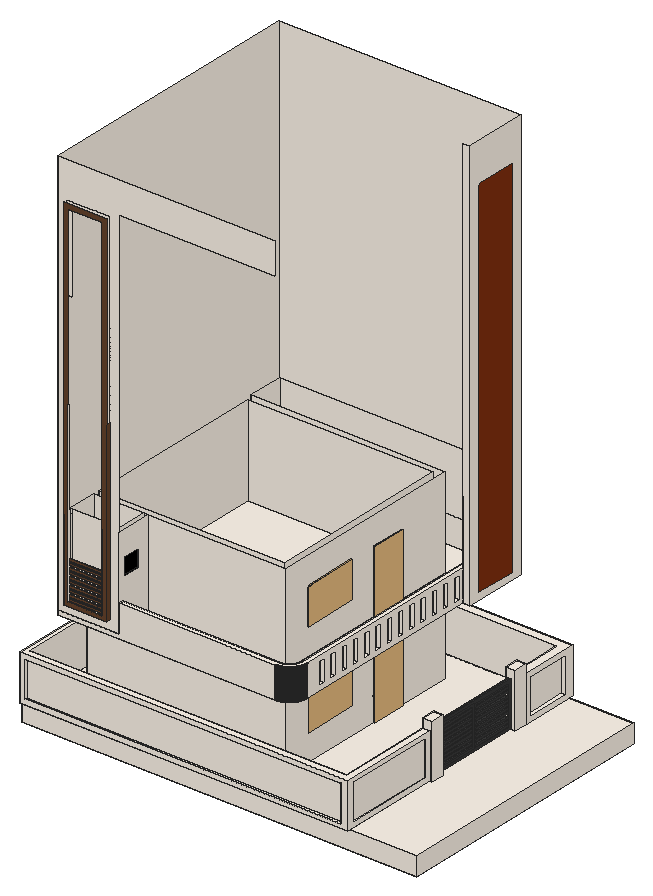
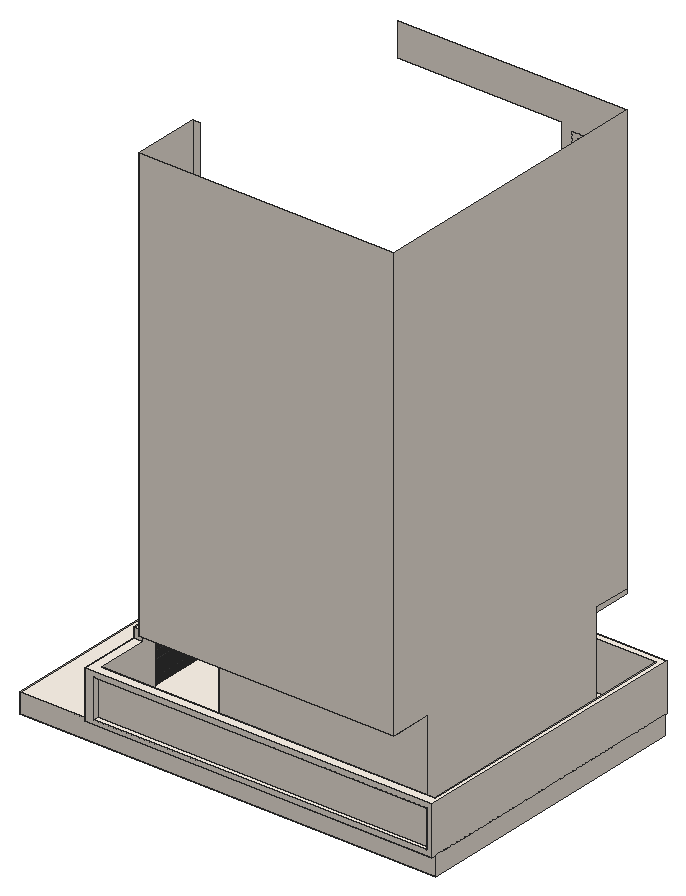
# SketchUp Ruby script. Lengths in inches.
U = 1.inch
M = Sketchup.active_model
def pt(a) = Geom::Point3d.new(a.map { |v| v * U })
def face(e, loops, mat)
  f = e.add_face(loops[0].map { |a| pt(a) })
  loops[1..].each { |l| e.add_face(l.map { |a| pt(a) }).erase! }
  f.material = f.back_material = mat if mat
  f
end
# faces: each face lists its corners as indices into pts; further lists are holes
def faces(e, pts, list, mat = nil) = list.each { |f| face(e, (f[0].is_a?(Array) ? f : [f]).map { |l| l.map { |i| pts[i] } }, mat) }
# xy, xz, yz: faces in a plane at the given z, y or x. An outline is a flat list of corners, or four numbers for a rectangle; further outlines are holes
def ring(l) = l.size == 4 ? [[l[0], l[1]], [l[2], l[1]], [l[2], l[3]], [l[0], l[3]]] : l.each_slice(2).to_a
def flat(e, list, mat, &to3) = list.each { |f| face(e, (f[0].is_a?(Array) ? f : [f]).map { |l| ring(l).map { |u, v| to3.(u, v) } }, mat) }
def xy(e, z, list, mat = nil) = flat(e, list, mat) { |x, y| [x, y, z] }
def xz(e, y, list, mat = nil) = flat(e, list, mat) { |x, z| [x, y, z] }
def yz(e, x, list, mat = nil) = flat(e, list, mat) { |y, z| [x, y, z] }
def lines(e, pts, list) = list.each { |a, b| e.add_line(pt(pts[a]), pt(pts[b])) }
# prism: a flat outline (further loops are holes) pulled along v
def prism(e, loops, v, mat = nil)
  f = face(e, loops, mat); d = Geom::Vector3d.new(v.map { |x| x * U })
  f.pushpull(f.normal.samedirection?(d) ? d.length : -d.length)
end
def box(e, o, s, mat = nil) = prism(e, [[o, [o[0] + s[0], o[1], o[2]], [o[0] + s[0], o[1] + s[1], o[2]], [o[0], o[1] + s[1], o[2]]]], [0, 0, s[2]], mat)
def at(x, y, z, deg = 0) = Geom::Transformation.translation(pt([x, y, z])) * Geom::Transformation.rotation(ORIGIN, Z_AXIS, deg.degrees)
def axes(o, x, y, z) = Geom::Transformation.new([*x, 0, *y, 0, *z, 0, *pt(o).to_a, 1])
def part(name) = M.definitions.add(name)
# library, detail: a bought-in or finely detailed component or shape, given as its bounding box
def library(name, o, s) = part(name).tap { |d| box(d.entities, o, s) }
def detail(e, o, s) = box(e.add_group.entities, o, s)
def put(e, d, t, mat = nil) = e.add_instance(d, t).tap { |i| i.material = mat if mat }
def group(e, t, mat = nil) = e.add_group.tap { |g| g.transformation = t; g.material = mat if mat }.entities
root = M.entities
M.materials.add("C01_Vanilla_Cream").color = [255, 246, 235]
M.materials.add("Hardwood_Double_Herringbone_4K").color = [130, 48, 16]
M.materials.add("M07_Charcoal_Gleam").color = [58, 58, 58]
M.materials.add("Wood_Veneer_15_1K").color = [103, 69, 45]
M.materials.add("[Color_009]1").color = [0, 0, 0]
c1 = library("porta+4",[0.2,-5.42,1.33],[46.55,4.72,83.21])
c2 = library("mesh-164",[-1582.71,-3144.16,-23.22],[2366.42,2227.34,65.81])
c3 = part("Group13")
put(c3.entities,c2,at(294.66,859.51,3.5))
xy(root,0,[[0,6,523.6875,366]],"C01_Vanilla_Cream")
xy(root,24,[[0,3,435,6],[[0,6,0,366,438,366,438,276.27,432,276.27,432,156.27,438,156.27,438,138.27,435,138.27,435,6],[6,12,426,12,426,156.27,429,156.27,429,276.27,426,276.27,426,360,6,360]],[435,6,523.6875,6,523.6875,366,438,366,438,276.27,432,276.27,432,156.27,438,156.27,438,138.27,435,138.27],[[6,12,426,12,426,156.27,429,156.27,429,276.27,426,276.27,426,360,6,360],[48,54,312,318]],[57,63,303,309],
  [0,366,438,372.04]],"C01_Vanilla_Cream")
xy(root,27,[[303,201,312,243]],"C01_Vanilla_Cream")
xy(root,30,[[6,3,426,6],[432,12,435,132.27],[432,300.27,438,360],[6,366,426,372.04]],"C01_Vanilla_Cream")
xy(root,31.5,[[429,161.27,432,214.27],[429,218.27,432,271.27]],"M07_Charcoal_Gleam")
xy(root,34,[[429,161.27,432,214.27],[429,218.27,432,271.27]],"C01_Vanilla_Cream")
xy(root,36.5,[[429,161.27,432,214.27],[429,218.27,432,271.27]],"M07_Charcoal_Gleam")
xy(root,39,[[429,218.27,432,271.27]],"C01_Vanilla_Cream")
xy(root,39,[[429,161.27,432,214.27]],"M07_Charcoal_Gleam")
xy(root,41.5,[[429,161.27,432,214.27],[429,218.27,432,271.27]],"M07_Charcoal_Gleam")
xy(root,44,[[429,218.27,432,271.27]],"C01_Vanilla_Cream")
xy(root,44,[[429,161.27,432,214.27]],"M07_Charcoal_Gleam")
xy(root,46.5,[[429,161.27,432,214.27],[429,218.27,432,271.27]],"M07_Charcoal_Gleam")
xy(root,49,[[429,161.27,432,214.27],[429,218.27,432,271.27]],"M07_Charcoal_Gleam")
xy(root,51.5,[[429,161.27,432,214.27],[429,218.27,432,271.27]],"M07_Charcoal_Gleam")
xy(root,54,[[429,161.27,432,214.27],[429,218.27,432,271.27]],"M07_Charcoal_Gleam")
xy(root,56.5,[[429,161.27,432,214.27],[429,218.27,432,271.27]],"M07_Charcoal_Gleam")
xy(root,59,[[429,161.27,432,214.27],[429,218.27,432,271.27]],"M07_Charcoal_Gleam")
xy(root,61.5,[[429,161.27,432,214.27],[429,218.27,432,271.27]],"M07_Charcoal_Gleam")
xy(root,63,[[303,93,312,159]],"C01_Vanilla_Cream")
xy(root,64,[[429,161.27,432,214.27],[429,218.27,432,271.27]],"M07_Charcoal_Gleam")
xy(root,66.5,[[429,161.27,432,214.27],[429,218.27,432,271.27]],"M07_Charcoal_Gleam")
xy(root,69,[[429,161.27,432,214.27],[429,218.27,432,271.27]],"M07_Charcoal_Gleam")
xy(root,71.5,[[429,161.27,432,214.27],[429,218.27,432,271.27]],"M07_Charcoal_Gleam")
xy(root,74,[[429,161.27,432,214.27],[429,218.27,432,271.27]],"M07_Charcoal_Gleam")
xy(root,76.5,[[429,161.27,432,214.27],[429,218.27,432,271.27]],"M07_Charcoal_Gleam")
xy(root,78,[[6,3,426,6],[432,12,435,132.27],[432,300.27,438,360],[6,366,426,372.04]],"C01_Vanilla_Cream")
xy(root,79,[[429,161.27,432,214.27],[429,218.27,432,271.27]],"M07_Charcoal_Gleam")
xy(root,84,[[0,3,435,3,435,138.27,426,138.27,426,12,6,12,6,360,426,360,426,294.27,438,294.27,438,372.04,0,372.04]],"C01_Vanilla_Cream")
xy(root,84,[[429,156.27,432,276.27]],"M07_Charcoal_Gleam")
xy(root,96,[[426,138.27,438,156.27],[426,276.27,438,294.27]],"C01_Vanilla_Cream")
xy(root,105,[[303,93,312,159],[303,201,312,243]],"C01_Vanilla_Cream")
xy(root,144,[[48,54,312,63],[57,63,303,309],[303,63,312,318],[360,288,360,366,48,366,48,372,369,372,369,288],[57,309,303,318],
  [48,318,57,366],[57,318,303,366],[303,318,312,366]],"C01_Vanilla_Cream")
xy(root,144,[[48,6,48,54,312,54,312,366,360,366,360,30,359.99,29.25,359.95,28.49,359.89,27.74,359.8125,26.99,359.7,26.25,359.57,25.5,359.42,24.76,359.25,24.03,359.05,23.3,358.83,22.58,358.58,21.87,358.31,21.17,358.03,20.47,357.72,19.78,357.38,19.1,357.03,18.4375,356.66,17.78,356.26,17.14,355.85,16.51,355.42,15.89,354.96,15.29,354.49,14.7,354,14.13,353.5,13.57,352.97,13.03,352.43,12.5,351.87,12,351.3,11.51,350.71,11.04,350.11,10.58,349.49,10.15,348.86,9.74,348.22,9.34,347.5625,8.97,346.9,8.62,346.22,8.28,345.53,7.97,344.83,7.69,344.13,7.42,343.42,7.17,342.7,6.95,341.97,6.75,341.24,6.58,340.5,6.43,339.75,6.3,339.01,6.1875,338.26,6.11,337.51,6.05,336.75,6.01,336,6]],"Wood_Veneer_15_1K")
xy(root,150,[[48,6,129,6,129,54,123,54,123,12,57,12,57,54,48,54],[129,12,336,12,336.57,12.01,337.13,12.04,337.69,12.08,338.26,12.14,338.82,12.22,339.37,12.32,339.93,12.43,340.48,12.57,341.02,12.71,341.5625,12.88,342.1,13.0625,342.625,13.26,343.15,13.48,343.66,13.71,344.17,13.96,344.67,14.23,345.16,14.51,345.64,14.8,346.12,15.11,346.58,15.4375,347.03,15.78,347.47,16.13,347.9,16.5,348.32,16.88,348.73,17.27,349.12,17.68,349.5,18.1,349.87,18.53,350.22,18.97,350.5625,19.42,350.89,19.88,351.2,20.36,351.49,20.84,351.77,21.33,352.04,21.83,352.29,22.34,352.52,22.85,352.74,23.375,352.9375,23.9,353.12,24.4375,353.29,24.98,353.43,25.52,353.57,26.07,353.68,26.63,353.78,27.18,353.86,27.74,353.92,28.31,353.96,28.87,353.99,29.43,354,30,354,366,54,366,54,318,312,318,312,54,129,54],[57,12,123,54],[354,48.59,360,57.93],[57,63,303,309],
  [354,67.26,360,76.6],[354,85.93,360,95.27],[354,104.61,360,113.94],[354,123.28,360,132.62],[354,141.95,360,151.29],
  [354,160.625,360,169.96],[354,179.3,360,188.64],[354,197.97,360,207.31],[354,216.64,360,225.98],[354,235.32,360,244.65],
  [354,253.99,360,263.33],[354,272.66,360,282]],"C01_Vanilla_Cream")
xy(root,153,[[303,201,312,243],[360,303,369,357]],"C01_Vanilla_Cream")
xy(root,162,[[60,0,117,6]],"Wood_Veneer_15_1K")
xy(root,168,[[66,0,111,6]],"C01_Vanilla_Cream")
xy(root,169,[[66,1,111,2]],"C01_Vanilla_Cream")
xy(root,171.68,[[66,1,111,2]],"C01_Vanilla_Cream")
xy(root,174.35,[[66,1,111,2]],"C01_Vanilla_Cream")
xy(root,177.03,[[66,1,111,2]],"C01_Vanilla_Cream")
xy(root,179.7,[[66,1,111,2]],"C01_Vanilla_Cream")
xy(root,180,[[354,48.59,360,57.93],[354,67.26,360,76.6],[354,85.93,360,95.27],[354,104.61,360,113.94],[354,123.28,360,132.62],
  [354,141.95,360,151.29],[354,160.625,360,169.96],[354,179.3,360,188.64],[354,197.97,360,207.31],[354,216.64,360,225.98],
  [354,235.32,360,244.65],[354,253.99,360,263.33],[354,272.66,360,282]],"C01_Vanilla_Cream")
xy(root,182.375,[[66,1,111,2]],"C01_Vanilla_Cream")
xy(root,185.05,[[66,1,111,2]],"C01_Vanilla_Cream")
xy(root,186,[[129,6,336,6,336.75,6.01,337.51,6.05,338.26,6.11,339.01,6.1875,339.75,6.3,340.5,6.43,341.24,6.58,341.97,6.75,342.7,6.95,343.42,7.17,344.13,7.42,344.83,7.69,345.53,7.97,346.22,8.28,346.9,8.62,347.5625,8.97,348.22,9.34,348.86,9.74,349.49,10.15,350.11,10.58,350.71,11.04,351.3,11.51,351.87,12,352.43,12.5,352.97,13.03,353.5,13.57,354,14.13,354.49,14.7,354.96,15.29,355.42,15.89,355.85,16.51,356.26,17.14,356.66,17.78,357.03,18.4375,357.38,19.1,357.72,19.78,358.03,20.47,358.31,21.17,358.58,21.87,358.83,22.58,359.05,23.3,359.25,24.03,359.42,24.76,359.57,25.5,359.7,26.25,359.8125,26.99,359.89,27.74,359.95,28.49,359.99,29.25,360,30,360,366,354,366,354,30,353.99,29.43,353.96,28.87,353.92,28.31,353.86,27.74,353.78,27.18,353.68,26.63,353.57,26.07,353.43,25.52,353.29,24.98,353.12,24.4375,352.9375,23.9,352.74,23.375,352.52,22.85,352.29,22.34,352.04,21.83,351.77,21.33,351.49,20.84,351.2,20.36,350.89,19.88,350.5625,19.42,350.22,18.97,349.87,18.53,349.5,18.1,349.12,17.68,348.73,17.27,348.32,16.88,347.9,16.5,347.47,16.13,347.03,15.78,346.58,15.4375,346.12,15.11,345.64,14.8,345.16,14.51,344.67,14.23,344.17,13.96,343.66,13.71,343.15,13.48,342.625,13.26,342.1,13.0625,341.5625,12.88,341.02,12.71,340.48,12.57,339.93,12.43,339.37,12.32,338.82,12.22,338.26,12.14,337.69,12.08,337.13,12.04,336.57,12.01,336,12,129,12]],"C01_Vanilla_Cream")
xy(root,187.73,[[66,1,111,2]],"C01_Vanilla_Cream")
xy(root,189,[[303,93,312,159]],"C01_Vanilla_Cream")
xy(root,190.4,[[66,1,111,2]],"C01_Vanilla_Cream")
xy(root,193.08,[[66,1,111,2]],"C01_Vanilla_Cream")
xy(root,195.75,[[66,1,111,2]],"C01_Vanilla_Cream")
xy(root,198.43,[[66,1,111,2]],"C01_Vanilla_Cream")
xy(root,201.1,[[66,1,111,2]],"C01_Vanilla_Cream")
xy(root,203.78,[[66,1,111,2]],"C01_Vanilla_Cream")
xy(root,206.45,[[66,1,111,2]],"C01_Vanilla_Cream")
xy(root,209.125,[[66,1,111,2]],"C01_Vanilla_Cream")
xy(root,211.8,[[66,1,111,2]],"C01_Vanilla_Cream")
xy(root,213.8,[[126,14.34,129,38.34]],"[Color_009]1")
xy(root,214.48,[[66,1,111,2]],"C01_Vanilla_Cream")
xy(root,217.15,[[66,1,111,2]],"C01_Vanilla_Cream")
xz(root,0,[[[60,162,117,642],[66,168,111,636]]],"Wood_Veneer_15_1K")
xz(root,1,[[66,169,111,171.68],[66,174.35,111,177.03],[66,179.7,111,182.375],[66,185.05,111,187.73],[66,190.4,111,193.08],
  [66,195.75,111,198.43],[66,201.1,111,203.78],[66,206.45,111,209.125],[66,211.8,111,214.48],[66,217.15,111,219.82]],"Wood_Veneer_15_1K")
xz(root,2,[[66,169,111,171.68],[66,174.35,111,177.03],[66,179.7,111,182.375],[66,185.05,111,187.73],[66,190.4,111,193.08],
  [66,195.75,111,198.43],[66,201.1,111,203.78],[66,206.45,111,209.125],[66,211.8,111,214.48],[66,217.15,111,219.82]],"C01_Vanilla_Cream")
xz(root,3,[[[0,24,435,84],[6,30,426,78]]],"C01_Vanilla_Cream")
xz(root,6,[[0,0,523.6875,24],[6,30,426,78],[48,144,336,144,336,186,129,186,129,150,48,150],[[48,150,129,150,129,648,336,648,336,690,48,690],[60,162,117,642]],[60,162,117,162,117,642,60,642,60,528,66,528,66,636,111,636,111,168,66,168,66,276,60,276],
  [66,168,111,276]],"C01_Vanilla_Cream")
xz(root,12,[[6,24,426,84],[432,30,435,78],[57,150,123,270],[129,150,135,186],[135,150,336,186]],"C01_Vanilla_Cream")
xz(root,14.34,[[126,213.8,129,237.8]],"[Color_009]1")
xz(root,38.34,[[126,213.8,129,237.8]],"[Color_009]1")
xz(root,48.59,[[354,150,360,180]],"C01_Vanilla_Cream")
xz(root,54,[[48,24,312,144],[48,144,57,150],[57,150,123,270],[123,150,129,270],[129,150,312,270]],"C01_Vanilla_Cream")
xz(root,57.93,[[354,150,360,180]],"C01_Vanilla_Cream")
xz(root,63,[[57,24,303,144],[57,150,303,270]],"C01_Vanilla_Cream")
xz(root,67.26,[[354,150,360,180]],"C01_Vanilla_Cream")
xz(root,76.6,[[354,150,360,180]],"C01_Vanilla_Cream")
xz(root,85.93,[[354,150,360,180]],"C01_Vanilla_Cream")
xz(root,93,[[303,63,312,105],[303,189,312,231]],"C01_Vanilla_Cream")
xz(root,95.27,[[354,150,360,180]],"C01_Vanilla_Cream")
xz(root,104.61,[[354,150,360,180]],"C01_Vanilla_Cream")
xz(root,113.94,[[354,150,360,180]],"C01_Vanilla_Cream")
xz(root,123.28,[[354,150,360,180]],"C01_Vanilla_Cream")
xz(root,132.27,[[432,30,435,78]],"C01_Vanilla_Cream")
xz(root,132.62,[[354,150,360,180]],"C01_Vanilla_Cream")
xz(root,138.27,[[435,24,438,24,438,96,426,96,426,84,435,84]],"C01_Vanilla_Cream")
xz(root,141.95,[[354,150,360,180]],"C01_Vanilla_Cream")
xz(root,151.29,[[354,150,360,180]],"C01_Vanilla_Cream")
xz(root,156.27,[[426,24,426,96,438,96,438,24,432,24,432,84,429,84,429,24]],"C01_Vanilla_Cream")
xz(root,159,[[303,63,312,105],[303,189,312,231]],"C01_Vanilla_Cream")
xz(root,160.625,[[354,150,360,180]],"C01_Vanilla_Cream")
xz(root,161.27,[[429,31.5,432,34],[429,36.5,432,39],[429,41.5,432,44],[429,46.5,432,49],[429,51.5,432,54],
  [429,56.5,432,59],[429,61.5,432,64],[429,66.5,432,69],[429,71.5,432,74],[429,76.5,432,79]],"C01_Vanilla_Cream")
xz(root,169.96,[[354,150,360,180]],"C01_Vanilla_Cream")
xz(root,179.3,[[354,150,360,180]],"C01_Vanilla_Cream")
xz(root,188.64,[[354,150,360,180]],"C01_Vanilla_Cream")
xz(root,197.97,[[354,150,360,180]],"C01_Vanilla_Cream")
xz(root,201,[[303,27,312,105],[303,153,312,231]],"C01_Vanilla_Cream")
xz(root,207.31,[[354,150,360,180]],"C01_Vanilla_Cream")
xz(root,214.27,[[429,31.5,432,34],[429,36.5,432,39],[429,41.5,432,44],[429,46.5,432,49],[429,51.5,432,54],
  [429,56.5,432,59],[429,61.5,432,64],[429,66.5,432,69],[429,71.5,432,74]],"C01_Vanilla_Cream")
xz(root,214.27,[[429,76.5,432,79]],"M07_Charcoal_Gleam")
xz(root,216.64,[[354,150,360,180]],"C01_Vanilla_Cream")
xz(root,218.27,[[429,31.5,432,34],[429,36.5,432,39],[429,41.5,432,44],[429,46.5,432,49],[429,51.5,432,54],
  [429,56.5,432,59],[429,61.5,432,64],[429,66.5,432,69],[429,71.5,432,74],[429,76.5,432,79]],"C01_Vanilla_Cream")
xz(root,225.98,[[354,150,360,180]],"C01_Vanilla_Cream")
xz(root,235.32,[[354,150,360,180]],"C01_Vanilla_Cream")
xz(root,243,[[303,27,312,105],[303,153,312,231]],"C01_Vanilla_Cream")
xz(root,244.65,[[354,150,360,180]],"C01_Vanilla_Cream")
xz(root,253.99,[[354,150,360,180]],"C01_Vanilla_Cream")
xz(root,263.33,[[354,150,360,180]],"C01_Vanilla_Cream")
xz(root,271.27,[[429,31.5,432,34],[429,36.5,432,39],[429,41.5,432,44],[429,46.5,432,49],[429,51.5,432,54],
  [429,56.5,432,59],[429,61.5,432,64],[429,66.5,432,69],[429,71.5,432,74],[429,76.5,432,79]],"C01_Vanilla_Cream")
xz(root,272.66,[[354,150,360,180]],"C01_Vanilla_Cream")
xz(root,276.27,[[426,24,429,24,429,84,432,84,432,24,438,24,438,96,426,96]],"C01_Vanilla_Cream")
xz(root,282,[[354,150,360,180]],"C01_Vanilla_Cream")
xz(root,288,[[360,144,369,690]],"C01_Vanilla_Cream")
xz(root,294.27,[[426,84,438,96]],"C01_Vanilla_Cream")
xz(root,300.27,[[432,30,438,78]],"C01_Vanilla_Cream")
xz(root,309,[[57,24,303,144],[57,150,303,270]],"C01_Vanilla_Cream")
xz(root,318,[[48,24,312,144],[54,150,312,270]],"C01_Vanilla_Cream")
xz(root,360,[[6,24,426,84],[432,30,438,78]],"C01_Vanilla_Cream")
xz(root,366,[[0,0,523.6875,24],[6,30,426,78],[54,150,354,186],[354,150,360,186],[54,186,360,270]],"C01_Vanilla_Cream")
xz(root,372,[[48,144,369,690]],"C01_Vanilla_Cream")
xz(root,372.04,[[[0,24,438,84],[6,30,426,78]]],"C01_Vanilla_Cream")
yz(root,0,[[6,0,366,24],[3,24,372.04,84]],"C01_Vanilla_Cream")
yz(root,6,[[12,24,360,84],[3,30,6,78],[366,30,372.04,78]],"C01_Vanilla_Cream")
yz(root,48,[[54,24,54,150,6,150,6,690,372,690,372,144,318,144,318,24],[6,144,54,150]],"C01_Vanilla_Cream")
yz(root,54,[[318,150,366,186],[318,186,366,270]],"C01_Vanilla_Cream")
yz(root,57,[[63,24,309,144],[12,150,54,270],[63,150,309,270]],"C01_Vanilla_Cream")
yz(root,60,[[0,162,6,270]],"Wood_Veneer_15_1K")
yz(root,66,[[0,168,3,168,3,276,2,276,2,169,1,169,1,402,0,402],[3,168,6,270],[1,171.68,2,174.35],[1,177.03,2,179.7],[1,182.375,2,185.05],
  [1,187.73,2,190.4],[1,193.08,2,195.75],[1,198.43,2,201.1],[1,203.78,2,206.45],[1,209.125,2,211.8],
  [1,214.48,2,217.15]],"C01_Vanilla_Cream")
yz(root,111,[[[0,168,6,270],[1,169,2,171.68],[1,179.7,2,182.375],[1,190.4,2,193.08],[1,201.1,2,203.78],[1,211.8,2,214.48],[1,249.25,2,251.92],[1,259.95,2,262.625],[1,265.3,2,267.98],[1,174.35,2,177.03],[1,185.05,2,187.73],[1,195.75,2,198.43],[1,206.45,2,209.125],[1,217.15,2,219.82],[1,222.5,2,225.17],[1,227.85,2,230.52],[1,233.2,2,235.875],[1,238.55,2,241.22],[1,243.9,2,246.58],[1,254.6,2,257.27]]],"C01_Vanilla_Cream")
yz(root,117,[[0,162,6,396]],"Wood_Veneer_15_1K")
yz(root,123,[[12,150,54,270]],"C01_Vanilla_Cream")
yz(root,126,[[14.34,213.8,38.34,237.8]],"[Color_009]1")
yz(root,129,[[6,150,12,186],[[12,150,54,150,54,270,6,270,6,186,12,186],[14.34,213.8,38.34,237.8]]],"C01_Vanilla_Cream")
yz(root,303,[[[63,24,309,144],[201,27,243,105],[93,63,159,105]],[[63,150,309,270],[201,153,243,231],[93,189,159,231]]],"C01_Vanilla_Cream")
yz(root,312,[[[54,24,198,24,198,108,246,108,246,24,318,24,318,144,54,144],[90,60,162,108]],[[198,24,246,108],[201,27,243,105]],[[90,60,162,108],[93,63,159,105]],[[54,150,198,150,198,234,246,234,246,150,318,150,318,270,54,270],[90,186,162,234]],[[198,150,246,234],[201,153,243,231]],
  [[90,186,162,234],[93,189,159,231]]],"C01_Vanilla_Cream")
yz(root,354,[[30,150,30,186,366,186,366,150,282,150,282,180,272.66,180,272.66,150,263.33,150,263.33,180,253.99,180,253.99,150,244.65,150,244.65,180,235.32,180,235.32,150,225.98,150,225.98,180,216.64,180,216.64,150,207.31,150,207.31,180,197.97,180,197.97,150,188.64,150,188.64,180,179.3,180,179.3,150,169.96,150,169.96,180,160.625,180,160.625,150,151.29,150,151.29,180,141.95,180,141.95,150,132.62,150,132.62,180,123.28,180,123.28,150,113.94,150,113.94,180,104.61,180,104.61,150,95.27,150,95.27,180,85.93,180,85.93,150,76.6,150,76.6,180,67.26,180,67.26,150,57.93,150,57.93,180,48.59,180,48.59,150]],"C01_Vanilla_Cream")
yz(root,360,[[[30,144,288,186],[48.59,150,57.93,180],[85.93,150,95.27,180],[104.61,150,113.94,180],[141.95,150,151.29,180],[123.28,150,132.62,180],[179.3,150,188.64,180],[216.64,150,225.98,180],[197.97,150,207.31,180],[253.99,150,263.33,180],[272.66,150,282,180],[67.26,150,76.6,180],[160.625,150,169.96,180],[235.32,150,244.65,180]],[288,144,366,150],[288,150,366,150,366,186,357,186,357,153,303,153,303,186,288,186],[303,153,357,186],[288,186,366,270]],"C01_Vanilla_Cream")
yz(root,369,[[[288,144,372,690],[303,153,357,639]]],"C01_Vanilla_Cream")
yz(root,369,[[303,153,357,639]],"Hardwood_Double_Herringbone_4K")
yz(root,426,[[12,24,12,84,138.27,84,138.27,96,156.27,96,156.27,24],[276.27,24,276.27,96,294.27,96,294.27,84,360,84,360,24],[3,30,6,78],[366,30,372.04,78]],"C01_Vanilla_Cream")
yz(root,429,[[[156.27,24,276.27,84],[161.27,76.5,214.27,79],[161.27,71.5,214.27,74],[161.27,66.5,214.27,69],[161.27,61.5,214.27,64],[161.27,56.5,214.27,59],[161.27,51.5,214.27,54],[161.27,46.5,214.27,49],[161.27,41.5,214.27,44],[161.27,36.5,214.27,39],[161.27,31.5,214.27,34],[218.27,76.5,271.27,79],[218.27,71.5,271.27,74],[218.27,66.5,271.27,69],[218.27,61.5,271.27,64],[218.27,56.5,271.27,59],[218.27,51.5,271.27,54],[218.27,46.5,271.27,49],[218.27,41.5,271.27,44],[218.27,36.5,271.27,39],[218.27,31.5,271.27,34]]],"M07_Charcoal_Gleam")
yz(root,432,[[12,30,132.27,78],[300.27,30,360,78]],"C01_Vanilla_Cream")
yz(root,432,[[[156.27,24,276.27,84],[159.27,27,273.27,81]],[[159.27,27,216.27,81],[161.27,29,214.27,79]],[[216.27,27,273.27,81],[218.27,29,271.27,79]],[161.27,29,214.27,31.5],[218.27,29,271.27,31.5],
  [161.27,34,214.27,36.5],[218.27,34,271.27,36.5],[161.27,39,214.27,41.5],[218.27,39,271.27,41.5],[161.27,44,214.27,46.5],
  [218.27,44,271.27,46.5],[161.27,49,214.27,51.5],[218.27,49,271.27,51.5],[161.27,54,214.27,56.5],[218.27,54,271.27,56.5],
  [161.27,59,214.27,61.5],[218.27,59,271.27,61.5],[161.27,64,214.27,66.5],[218.27,64,271.27,66.5],[161.27,69,214.27,71.5],
  [218.27,69,271.27,71.5],[161.27,74,214.27,76.5],[218.27,74,271.27,76.5]],"M07_Charcoal_Gleam")
yz(root,435,[[[3,24,138.27,84],[12,30,132.27,78]]],"C01_Vanilla_Cream")
yz(root,438,[[138.27,24,156.27,96],[276.27,24,294.27,96],[[294.27,24,372.04,84],[300.27,30,360,78]]],"C01_Vanilla_Cream")
yz(root,523.6875,[[6,0,366,24]],"C01_Vanilla_Cream")
p = [[336.75,6.01,144],[336.75,6.01,186],[336,6,186],[336,6,144],[337.51,6.05,144],[337.51,6.05,186],
  [338.26,6.11,144],[338.26,6.11,186],[339.01,6.1875,144],[339.01,6.1875,186],[339.75,6.3,144],[339.75,6.3,186],
  [340.5,6.43,144],[340.5,6.43,186],[341.24,6.58,144],[341.24,6.58,186],[341.97,6.75,144],[341.97,6.75,186],
  [342.7,6.95,144],[342.7,6.95,186],[343.42,7.17,144],[343.42,7.17,186],[344.13,7.42,144],[344.13,7.42,186],
  [344.83,7.69,144],[344.83,7.69,186],[345.53,7.97,144],[345.53,7.97,186],[346.22,8.28,144],[346.22,8.28,186],
  [346.9,8.62,144],[346.9,8.62,186],[347.5625,8.97,144],[347.5625,8.97,186],[348.22,9.34,144],[348.22,9.34,186],
  [348.86,9.74,144],[348.86,9.74,186],[349.49,10.15,144],[349.49,10.15,186],[350.11,10.58,144],[350.11,10.58,186],
  [350.71,11.04,144],[350.71,11.04,186],[351.3,11.51,144],[351.3,11.51,186],[351.87,12,144],[351.87,12,186],
  [352.43,12.5,144],[352.43,12.5,186],[352.97,13.03,144],[352.97,13.03,186],[353.5,13.57,144],[353.5,13.57,186],
  [354,14.13,144],[354,14.13,186],[354.49,14.7,144],[354.49,14.7,186],[354.96,15.29,144],[354.96,15.29,186],
  [355.42,15.89,144],[355.42,15.89,186],[355.85,16.51,144],[355.85,16.51,186],[356.26,17.14,144],[356.26,17.14,186],
  [356.66,17.78,144],[356.66,17.78,186],[357.03,18.4375,144],[357.03,18.4375,186],[357.38,19.1,144],[357.38,19.1,186],
  [357.72,19.78,144],[357.72,19.78,186],[358.03,20.47,144],[358.03,20.47,186],[358.31,21.17,144],[358.31,21.17,186],
  [358.58,21.87,144],[358.58,21.87,186],[358.83,22.58,144],[358.83,22.58,186],[359.05,23.3,144],[359.05,23.3,186],
  [359.25,24.03,144],[359.25,24.03,186],[359.42,24.76,144],[359.42,24.76,186],[359.57,25.5,144],[359.57,25.5,186],
  [359.7,26.25,144],[359.7,26.25,186],[359.8125,26.99,144],[359.8125,26.99,186],[359.89,27.74,144],[359.89,27.74,186],
  [359.95,28.49,144],[359.95,28.49,186],[359.99,29.25,144],[359.99,29.25,186],[360,30,144],[360,30,186],
  [336.57,12.01,150],[336,12,150],[336,12,186],[336.57,12.01,186],[337.13,12.04,150],[337.13,12.04,186],
  [337.69,12.08,150],[337.69,12.08,186],[338.26,12.14,150],[338.26,12.14,186],[338.82,12.22,150],[338.82,12.22,186],
  [339.37,12.32,150],[339.37,12.32,186],[339.93,12.43,150],[339.93,12.43,186],[340.48,12.57,150],[340.48,12.57,186],
  [341.02,12.71,150],[341.02,12.71,186],[341.5625,12.88,150],[341.5625,12.88,186],[342.1,13.0625,150],[342.1,13.0625,186],
  [342.625,13.26,150],[342.625,13.26,186],[343.15,13.48,150],[343.15,13.48,186],[343.66,13.71,150],[343.66,13.71,186],
  [344.17,13.96,150],[344.17,13.96,186],[344.67,14.23,150],[344.67,14.23,186],[345.16,14.51,150],[345.16,14.51,186],
  [345.64,14.8,150],[345.64,14.8,186],[346.12,15.11,150],[346.12,15.11,186],[346.58,15.4375,150],[346.58,15.4375,186],
  [347.03,15.78,150],[347.03,15.78,186],[347.47,16.13,150],[347.47,16.13,186],[347.9,16.5,150],[347.9,16.5,186],
  [348.32,16.88,150],[348.32,16.88,186],[348.73,17.27,150],[348.73,17.27,186],[349.12,17.68,150],[349.12,17.68,186],
  [349.5,18.1,150],[349.5,18.1,186],[349.87,18.53,150],[349.87,18.53,186],[350.22,18.97,150],[350.22,18.97,186],
  [350.5625,19.42,150],[350.5625,19.42,186],[350.89,19.88,150],[350.89,19.88,186],[351.2,20.36,150],[351.2,20.36,186],
  [351.49,20.84,150],[351.49,20.84,186],[351.77,21.33,150],[351.77,21.33,186],[352.04,21.83,150],[352.04,21.83,186],
  [352.29,22.34,150],[352.29,22.34,186],[352.52,22.85,150],[352.52,22.85,186],[352.74,23.375,150],[352.74,23.375,186],
  [352.9375,23.9,150],[352.9375,23.9,186],[353.12,24.4375,150],[353.12,24.4375,186],[353.29,24.98,150],[353.29,24.98,186],
  [353.43,25.52,150],[353.43,25.52,186],[353.57,26.07,150],[353.57,26.07,186],[353.68,26.63,150],[353.68,26.63,186],
  [353.78,27.18,150],[353.78,27.18,186],[353.86,27.74,150],[353.86,27.74,186],[353.92,28.31,150],[353.92,28.31,186],
  [353.96,28.87,150],[353.96,28.87,186],[353.99,29.43,150],[353.99,29.43,186],[354,30,150],[354,30,186],
  [57,12,150],[57,12,144],[129,12,150],[129,12,144],[135,48,150],[135,12,150],
  [54,318,150],[48,318,150]]
faces(root,p,[[0,1,2,3],[4,5,1,0],[6,7,5,4],[8,9,7,6],[10,11,9,8],[12,13,11,10],[14,15,13,12],[16,17,15,14],
  [18,19,17,16],[20,21,19,18],[22,23,21,20],[24,25,23,22],[26,27,25,24],[28,29,27,26],[30,31,29,28],[32,33,31,30],
  [34,35,33,32],[36,37,35,34],[38,39,37,36],[40,41,39,38],[42,43,41,40],[44,45,43,42],[46,47,45,44],[48,49,47,46],
  [50,51,49,48],[52,53,51,50],[54,55,53,52],[56,57,55,54],[58,59,57,56],[60,61,59,58],[62,63,61,60],[64,65,63,62],
  [66,67,65,64],[68,69,67,66],[70,71,69,68],[72,73,71,70],[74,75,73,72],[76,77,75,74],[78,79,77,76],[80,81,79,78],
  [82,83,81,80],[84,85,83,82],[86,87,85,84],[88,89,87,86],[90,91,89,88],[92,93,91,90],[94,95,93,92],[96,97,95,94],
  [98,99,97,96],[100,101,99,98],[102,103,104,105],[106,102,105,107],[108,106,107,109],[110,108,109,111],[112,110,111,113],[114,112,113,115],
  [116,114,115,117],[118,116,117,119],[120,118,119,121],[122,120,121,123],[124,122,123,125],[126,124,125,127],[128,126,127,129],[130,128,129,131],
  [132,130,131,133],[134,132,133,135],[136,134,135,137],[138,136,137,139],[140,138,139,141],[142,140,141,143],[144,142,143,145],[146,144,145,147],
  [148,146,147,149],[150,148,149,151],[152,150,151,153],[154,152,153,155],[156,154,155,157],[158,156,157,159],[160,158,159,161],[162,160,161,163],
  [164,162,163,165],[166,164,165,167],[168,166,167,169],[170,168,169,171],[172,170,171,173],[174,172,173,175],[176,174,175,177],[178,176,177,179],
  [180,178,179,181],[182,180,181,183],[184,182,183,185],[186,184,185,187],[188,186,187,189],[190,188,189,191],[192,190,191,193],[194,192,193,195],
  [196,194,195,197],[198,196,197,199],[200,198,199,201],[202,200,201,203]],"C01_Vanilla_Cream")
lines(root,p,[[204,205],[206,207],[208,209],[210,211]])
put(root,c1,at(309.24,197.8,23.48,90))
put(root,c3,axes([312.38,129.14,109.23],[0,0.03051,0],[0,0,0.02146],[0.01969,0,0]))
put(root,c1,at(309.24,197.8,149.48,90))
put(root,c3,axes([312.39,129.3,235.23],[0,0.03051,0],[0,0,0.02146],[0.01969,0,0]))
